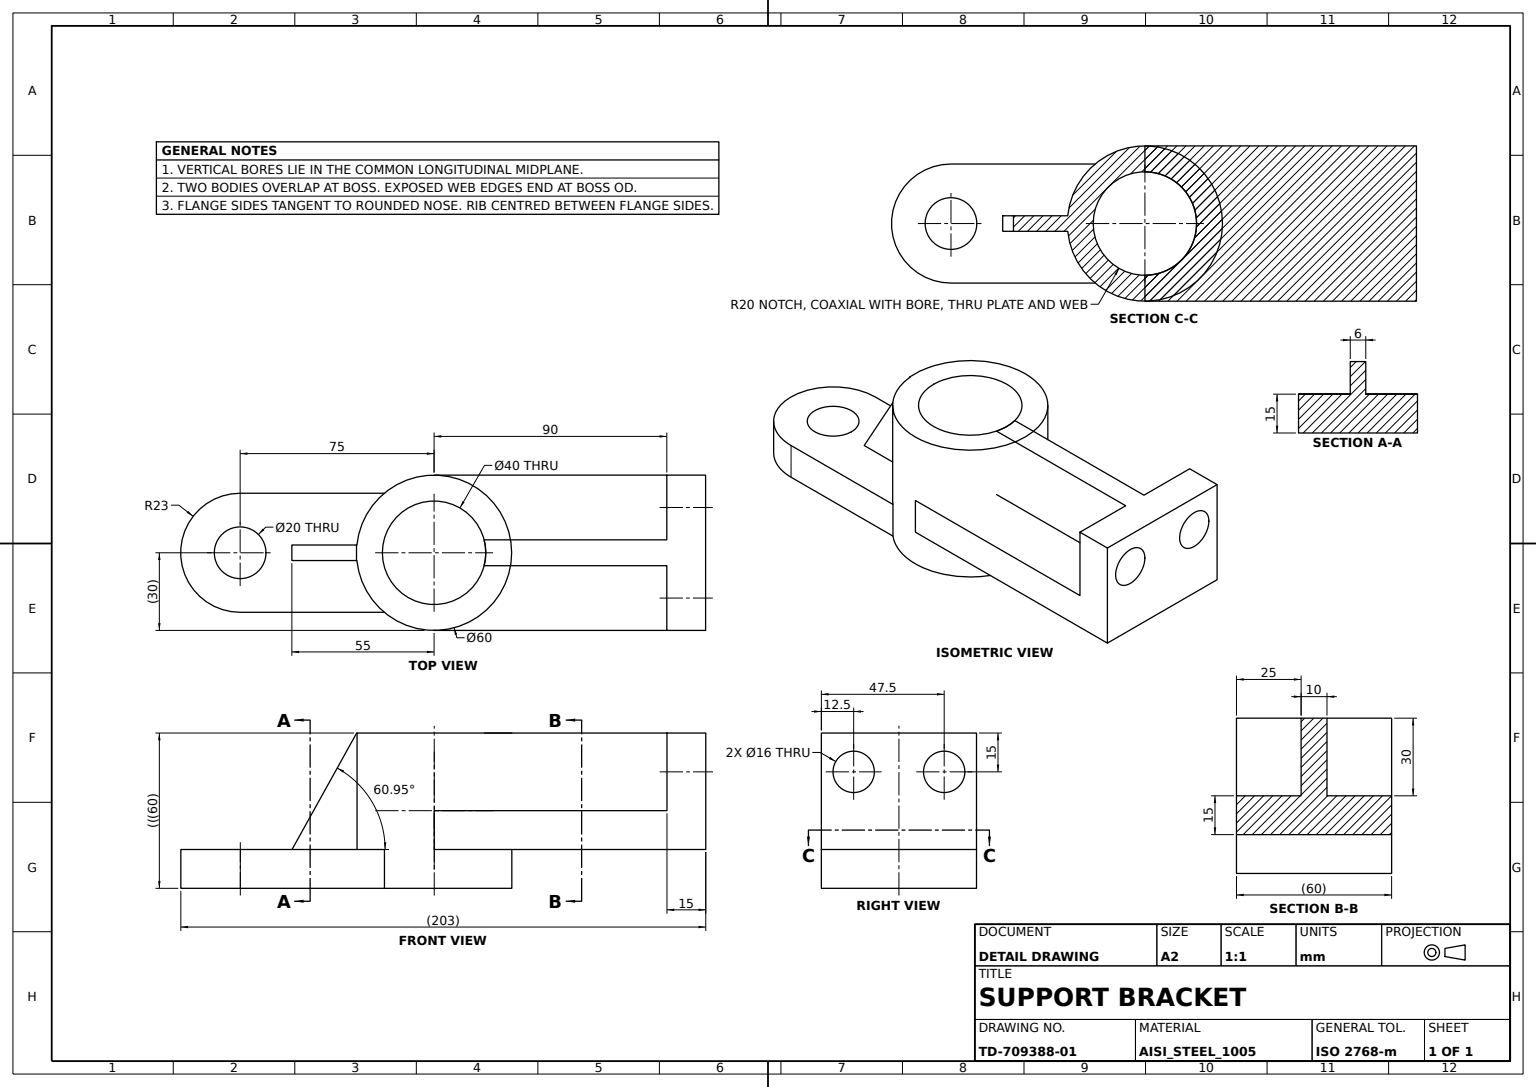
ISO-10303-21;
HEADER;
FILE_DESCRIPTION((''),'2;1');
FILE_NAME('','',(''),(''),'','','');
FILE_SCHEMA(('AUTOMOTIVE_DESIGN'));
ENDSEC;
DATA;
#1=APPLICATION_CONTEXT('');
#2=PRODUCT_CONTEXT('',#1,'mechanical');
#3=PRODUCT('','','',(#2));
#4=PRODUCT_DEFINITION_FORMATION('','',#3);
#5=PRODUCT_DEFINITION_CONTEXT('',#1,'design');
#6=PRODUCT_DEFINITION('','',#4,#5);
#7=PRODUCT_DEFINITION_SHAPE('','',#6);
#8=(LENGTH_UNIT()NAMED_UNIT(*)SI_UNIT(.MILLI.,.METRE.));
#9=(NAMED_UNIT(*)PLANE_ANGLE_UNIT()SI_UNIT($,.RADIAN.));
#10=(NAMED_UNIT(*)SI_UNIT($,.STERADIAN.)SOLID_ANGLE_UNIT());
#11=UNCERTAINTY_MEASURE_WITH_UNIT(LENGTH_MEASURE(0.005),#8,'distance_accuracy_value','');
#12=(GEOMETRIC_REPRESENTATION_CONTEXT(3)GLOBAL_UNCERTAINTY_ASSIGNED_CONTEXT((#11))GLOBAL_UNIT_ASSIGNED_CONTEXT((#8,#9,#10))REPRESENTATION_CONTEXT('',''));
#13=CARTESIAN_POINT('',(85.,0.,0.));
#14=VERTEX_POINT('',#13);
#15=CARTESIAN_POINT('',(75.,0.,0.));
#16=DIRECTION('',(0.,0.,1.));
#17=DIRECTION('',(1.,0.,0.));
#18=AXIS2_PLACEMENT_3D('',#15,#16,#17);
#19=CIRCLE('',#18,10.);
#20=EDGE_CURVE('',#14,#14,#19,.T.);
#21=ORIENTED_EDGE('',*,*,#20,.T.);
#22=EDGE_LOOP('',(#21));
#23=FACE_BOUND('',#22,.T.);
#24=CARTESIAN_POINT('',(20.,0.,0.));
#25=VERTEX_POINT('',#24);
#26=CARTESIAN_POINT('',(0.,0.,0.));
#27=AXIS2_PLACEMENT_3D('',#26,#16,#17);
#28=CIRCLE('',#27,20.);
#29=EDGE_CURVE('',#25,#25,#28,.T.);
#30=ORIENTED_EDGE('',*,*,#29,.T.);
#31=EDGE_LOOP('',(#30));
#32=FACE_BOUND('',#31,.T.);
#33=CARTESIAN_POINT('',(19.26136,-23.,0.));
#34=VERTEX_POINT('',#33);
#35=CARTESIAN_POINT('',(75.,-23.,0.));
#36=VERTEX_POINT('',#35);
#37=VECTOR('',#17,1000.);
#38=LINE('',#33,#37);
#39=EDGE_CURVE('',#34,#36,#38,.T.);
#40=ORIENTED_EDGE('',*,*,#39,.F.);
#41=CARTESIAN_POINT('',(19.26136,23.,0.));
#42=VERTEX_POINT('',#41);
#43=CIRCLE('',#27,30.);
#44=EDGE_CURVE('',#42,#34,#43,.T.);
#45=ORIENTED_EDGE('',*,*,#44,.F.);
#46=CARTESIAN_POINT('',(75.,23.,0.));
#47=VERTEX_POINT('',#46);
#48=DIRECTION('',(-1.,0.,0.));
#49=VECTOR('',#48,1000.);
#50=LINE('',#46,#49);
#51=EDGE_CURVE('',#47,#42,#50,.T.);
#52=ORIENTED_EDGE('',*,*,#51,.F.);
#53=CIRCLE('',#18,23.);
#54=EDGE_CURVE('',#36,#47,#53,.T.);
#55=ORIENTED_EDGE('',*,*,#54,.F.);
#56=EDGE_LOOP('',(#40,#45,#52,#55));
#57=FACE_BOUND('',#56,.T.);
#58=PLANE('',#27);
#59=ADVANCED_FACE('',(#23,#32,#57),#58,.F.);
#60=CARTESIAN_POINT('',(75.,23.,15.));
#61=VERTEX_POINT('',#60);
#62=DIRECTION('',(0.,0.,-1.));
#63=VECTOR('',#62,1000.);
#64=LINE('',#60,#63);
#65=EDGE_CURVE('',#61,#47,#64,.T.);
#66=ORIENTED_EDGE('',*,*,#65,.T.);
#67=ORIENTED_EDGE('',*,*,#51,.T.);
#68=CARTESIAN_POINT('',(19.26136,23.,15.));
#69=VERTEX_POINT('',#68);
#70=LINE('',#68,#63);
#71=EDGE_CURVE('',#69,#42,#70,.T.);
#72=ORIENTED_EDGE('',*,*,#71,.F.);
#73=LINE('',#60,#49);
#74=EDGE_CURVE('',#61,#69,#73,.T.);
#75=ORIENTED_EDGE('',*,*,#74,.F.);
#76=EDGE_LOOP('',(#66,#67,#72,#75));
#77=FACE_BOUND('',#76,.T.);
#78=DIRECTION('',(0.,-1.,0.));
#79=AXIS2_PLACEMENT_3D('',#60,#78,#62);
#80=PLANE('',#79);
#81=ADVANCED_FACE('',(#77),#80,.F.);
#82=CARTESIAN_POINT('',(29.849623,3.,15.));
#83=VERTEX_POINT('',#82);
#84=CARTESIAN_POINT('',(55.,3.,15.));
#85=VERTEX_POINT('',#84);
#86=CARTESIAN_POINT('',(0.,3.,15.));
#87=LINE('',#86,#49);
#88=EDGE_CURVE('',#83,#85,#87,.F.);
#89=ORIENTED_EDGE('',*,*,#88,.F.);
#90=CARTESIAN_POINT('',(29.849623,3.,60.));
#91=VERTEX_POINT('',#90);
#92=LINE('',#90,#63);
#93=EDGE_CURVE('',#91,#83,#92,.T.);
#94=ORIENTED_EDGE('',*,*,#93,.F.);
#95=CARTESIAN_POINT('',(30.,3.,60.));
#96=VERTEX_POINT('',#95);
#97=CARTESIAN_POINT('',(26.5,3.,60.));
#98=LINE('',#97,#37);
#99=EDGE_CURVE('',#91,#96,#98,.T.);
#100=ORIENTED_EDGE('',*,*,#99,.T.);
#101=DIRECTION('',(0.485642931,0.,-0.874157276));
#102=VECTOR('',#101,1000.);
#103=LINE('',#95,#102);
#104=EDGE_CURVE('',#96,#85,#103,.T.);
#105=ORIENTED_EDGE('',*,*,#104,.T.);
#106=EDGE_LOOP('',(#89,#94,#100,#105));
#107=FACE_BOUND('',#106,.T.);
#108=CARTESIAN_POINT('',(0.,3.,0.));
#109=DIRECTION('',(0.,1.,0.));
#110=AXIS2_PLACEMENT_3D('',#108,#109,#16);
#111=PLANE('',#110);
#112=ADVANCED_FACE('',(#107),#111,.T.);
#113=CARTESIAN_POINT('',(29.849623,-3.,15.));
#114=VERTEX_POINT('',#113);
#115=CARTESIAN_POINT('',(29.849623,-3.,60.));
#116=VERTEX_POINT('',#115);
#117=LINE('',#115,#63);
#118=EDGE_CURVE('',#114,#116,#117,.F.);
#119=ORIENTED_EDGE('',*,*,#118,.F.);
#120=CARTESIAN_POINT('',(55.,-3.,15.));
#121=VERTEX_POINT('',#120);
#122=CARTESIAN_POINT('',(0.,-3.,15.));
#123=LINE('',#122,#49);
#124=EDGE_CURVE('',#121,#114,#123,.T.);
#125=ORIENTED_EDGE('',*,*,#124,.F.);
#126=CARTESIAN_POINT('',(30.,-3.,60.));
#127=VERTEX_POINT('',#126);
#128=LINE('',#126,#102);
#129=EDGE_CURVE('',#127,#121,#128,.T.);
#130=ORIENTED_EDGE('',*,*,#129,.F.);
#131=CARTESIAN_POINT('',(26.5,-3.,60.));
#132=LINE('',#131,#37);
#133=EDGE_CURVE('',#116,#127,#132,.T.);
#134=ORIENTED_EDGE('',*,*,#133,.F.);
#135=EDGE_LOOP('',(#119,#125,#130,#134));
#136=FACE_BOUND('',#135,.T.);
#137=CARTESIAN_POINT('',(0.,-3.,0.));
#138=AXIS2_PLACEMENT_3D('',#137,#109,#16);
#139=PLANE('',#138);
#140=ADVANCED_FACE('',(#136),#139,.F.);
#141=VECTOR('',#109,1000.);
#142=LINE('',#126,#141);
#143=EDGE_CURVE('',#127,#96,#142,.T.);
#144=ORIENTED_EDGE('',*,*,#143,.T.);
#145=ORIENTED_EDGE('',*,*,#99,.F.);
#146=CARTESIAN_POINT('',(0.,0.,60.));
#147=AXIS2_PLACEMENT_3D('',#146,#16,#17);
#148=CIRCLE('',#147,30.);
#149=EDGE_CURVE('',#91,#116,#148,.T.);
#150=ORIENTED_EDGE('',*,*,#149,.T.);
#151=ORIENTED_EDGE('',*,*,#133,.T.);
#152=EDGE_LOOP('',(#144,#145,#150,#151));
#153=FACE_BOUND('',#152,.T.);
#154=CARTESIAN_POINT('',(20.,0.,60.));
#155=VERTEX_POINT('',#154);
#156=CIRCLE('',#147,20.);
#157=EDGE_CURVE('',#155,#155,#156,.T.);
#158=ORIENTED_EDGE('',*,*,#157,.F.);
#159=EDGE_LOOP('',(#158));
#160=FACE_BOUND('',#159,.T.);
#161=PLANE('',#147);
#162=ADVANCED_FACE('',(#153,#160),#161,.T.);
#163=CARTESIAN_POINT('',(75.,-23.,15.));
#164=VERTEX_POINT('',#163);
#165=LINE('',#163,#63);
#166=EDGE_CURVE('',#164,#36,#165,.T.);
#167=ORIENTED_EDGE('',*,*,#166,.F.);
#168=CARTESIAN_POINT('',(19.26136,-23.,15.));
#169=VERTEX_POINT('',#168);
#170=LINE('',#168,#37);
#171=EDGE_CURVE('',#169,#164,#170,.T.);
#172=ORIENTED_EDGE('',*,*,#171,.F.);
#173=LINE('',#168,#63);
#174=EDGE_CURVE('',#169,#34,#173,.T.);
#175=ORIENTED_EDGE('',*,*,#174,.T.);
#176=ORIENTED_EDGE('',*,*,#39,.T.);
#177=EDGE_LOOP('',(#167,#172,#175,#176));
#178=FACE_BOUND('',#177,.T.);
#179=AXIS2_PLACEMENT_3D('',#168,#109,#16);
#180=PLANE('',#179);
#181=ADVANCED_FACE('',(#178),#180,.F.);
#182=ORIENTED_EDGE('',*,*,#54,.T.);
#183=ORIENTED_EDGE('',*,*,#65,.F.);
#184=CARTESIAN_POINT('',(75.,0.,15.));
#185=AXIS2_PLACEMENT_3D('',#184,#16,#17);
#186=CIRCLE('',#185,23.);
#187=EDGE_CURVE('',#164,#61,#186,.T.);
#188=ORIENTED_EDGE('',*,*,#187,.F.);
#189=ORIENTED_EDGE('',*,*,#166,.T.);
#190=EDGE_LOOP('',(#182,#183,#188,#189));
#191=FACE_BOUND('',#190,.T.);
#192=AXIS2_PLACEMENT_3D('',#184,#62,#48);
#193=CYLINDRICAL_SURFACE('',#192,23.);
#194=ADVANCED_FACE('',(#191),#193,.T.);
#195=CARTESIAN_POINT('',(0.,0.,15.));
#196=AXIS2_PLACEMENT_3D('',#195,#62,#17);
#197=CIRCLE('',#196,30.);
#198=EDGE_CURVE('',#69,#83,#197,.T.);
#199=ORIENTED_EDGE('',*,*,#198,.F.);
#200=ORIENTED_EDGE('',*,*,#71,.T.);
#201=ORIENTED_EDGE('',*,*,#44,.T.);
#202=ORIENTED_EDGE('',*,*,#174,.F.);
#203=EDGE_CURVE('',#114,#169,#197,.T.);
#204=ORIENTED_EDGE('',*,*,#203,.F.);
#205=ORIENTED_EDGE('',*,*,#118,.T.);
#206=ORIENTED_EDGE('',*,*,#149,.F.);
#207=ORIENTED_EDGE('',*,*,#93,.T.);
#208=EDGE_LOOP('',(#199,#200,#201,#202,#204,#205,#206,#207));
#209=FACE_BOUND('',#208,.T.);
#210=AXIS2_PLACEMENT_3D('',#146,#62,#48);
#211=CYLINDRICAL_SURFACE('',#210,30.);
#212=ADVANCED_FACE('',(#209),#211,.T.);
#213=ORIENTED_EDGE('',*,*,#157,.T.);
#214=EDGE_LOOP('',(#213));
#215=FACE_BOUND('',#214,.T.);
#216=ORIENTED_EDGE('',*,*,#29,.F.);
#217=EDGE_LOOP('',(#216));
#218=FACE_BOUND('',#217,.T.);
#219=CYLINDRICAL_SURFACE('',#210,20.);
#220=ADVANCED_FACE('',(#215,#218),#219,.F.);
#221=ORIENTED_EDGE('',*,*,#20,.F.);
#222=EDGE_LOOP('',(#221));
#223=FACE_BOUND('',#222,.T.);
#224=CARTESIAN_POINT('',(65.,0.,15.));
#225=VERTEX_POINT('',#224);
#226=CIRCLE('',#192,10.);
#227=EDGE_CURVE('',#225,#225,#226,.F.);
#228=ORIENTED_EDGE('',*,*,#227,.T.);
#229=EDGE_LOOP('',(#228));
#230=FACE_BOUND('',#229,.T.);
#231=CARTESIAN_POINT('',(75.,0.,60.));
#232=AXIS2_PLACEMENT_3D('',#231,#62,#48);
#233=CYLINDRICAL_SURFACE('',#232,10.);
#234=ADVANCED_FACE('',(#223,#230),#233,.F.);
#235=ORIENTED_EDGE('',*,*,#203,.T.);
#236=ORIENTED_EDGE('',*,*,#171,.T.);
#237=ORIENTED_EDGE('',*,*,#187,.T.);
#238=ORIENTED_EDGE('',*,*,#74,.T.);
#239=ORIENTED_EDGE('',*,*,#198,.T.);
#240=ORIENTED_EDGE('',*,*,#88,.T.);
#241=LINE('',#120,#141);
#242=EDGE_CURVE('',#85,#121,#241,.F.);
#243=ORIENTED_EDGE('',*,*,#242,.T.);
#244=ORIENTED_EDGE('',*,*,#124,.T.);
#245=EDGE_LOOP('',(#235,#236,#237,#238,#239,#240,#243,#244));
#246=FACE_BOUND('',#245,.T.);
#247=ORIENTED_EDGE('',*,*,#227,.F.);
#248=EDGE_LOOP('',(#247));
#249=FACE_BOUND('',#248,.T.);
#250=AXIS2_PLACEMENT_3D('',#195,#62,#48);
#251=PLANE('',#250);
#252=ADVANCED_FACE('',(#246,#249),#251,.F.);
#253=ORIENTED_EDGE('',*,*,#143,.F.);
#254=ORIENTED_EDGE('',*,*,#129,.T.);
#255=ORIENTED_EDGE('',*,*,#242,.F.);
#256=ORIENTED_EDGE('',*,*,#104,.F.);
#257=EDGE_LOOP('',(#253,#254,#255,#256));
#258=FACE_BOUND('',#257,.T.);
#259=DIRECTION('',(0.874157276,0.,0.485642931));
#260=AXIS2_PLACEMENT_3D('',#126,#259,#101);
#261=PLANE('',#260);
#262=ADVANCED_FACE('',(#258),#261,.T.);
#263=CLOSED_SHELL('',(#59,#81,#112,#140,#162,#181,#194,#212,#220,#234,#252,#262));
#264=MANIFOLD_SOLID_BREP('',#263);
#265=CARTESIAN_POINT('',(-90.,5.,60.));
#266=VERTEX_POINT('',#265);
#267=CARTESIAN_POINT('',(-90.,30.,60.));
#268=VERTEX_POINT('',#267);
#269=CARTESIAN_POINT('',(-90.,-30.,60.));
#270=LINE('',#269,#141);
#271=EDGE_CURVE('',#266,#268,#270,.T.);
#272=ORIENTED_EDGE('',*,*,#271,.F.);
#273=CARTESIAN_POINT('',(-90.,5.,30.));
#274=VERTEX_POINT('',#273);
#275=LINE('',#265,#63);
#276=EDGE_CURVE('',#266,#274,#275,.T.);
#277=ORIENTED_EDGE('',*,*,#276,.T.);
#278=CARTESIAN_POINT('',(-90.,30.,30.));
#279=VERTEX_POINT('',#278);
#280=CARTESIAN_POINT('',(-90.,-30.,30.));
#281=LINE('',#280,#141);
#282=EDGE_CURVE('',#274,#279,#281,.T.);
#283=ORIENTED_EDGE('',*,*,#282,.T.);
#284=VECTOR('',#16,1000.);
#285=LINE('',#278,#284);
#286=EDGE_CURVE('',#279,#268,#285,.T.);
#287=ORIENTED_EDGE('',*,*,#286,.T.);
#288=EDGE_LOOP('',(#272,#277,#283,#287));
#289=FACE_BOUND('',#288,.T.);
#290=CARTESIAN_POINT('',(-90.,17.5,53.));
#291=VERTEX_POINT('',#290);
#292=CARTESIAN_POINT('',(-90.,17.5,45.));
#293=AXIS2_PLACEMENT_3D('',#292,#48,#16);
#294=CIRCLE('',#293,8.);
#295=EDGE_CURVE('',#291,#291,#294,.T.);
#296=ORIENTED_EDGE('',*,*,#295,.T.);
#297=EDGE_LOOP('',(#296));
#298=FACE_BOUND('',#297,.T.);
#299=AXIS2_PLACEMENT_3D('',#280,#48,#16);
#300=PLANE('',#299);
#301=ADVANCED_FACE('',(#289,#298),#300,.F.);
#302=CARTESIAN_POINT('',(0.,20.,30.));
#303=VERTEX_POINT('',#302);
#304=CARTESIAN_POINT('',(0.,30.,30.));
#305=VERTEX_POINT('',#304);
#306=CARTESIAN_POINT('',(0.,-30.,30.));
#307=LINE('',#306,#141);
#308=EDGE_CURVE('',#303,#305,#307,.T.);
#309=ORIENTED_EDGE('',*,*,#308,.F.);
#310=CARTESIAN_POINT('',(0.,20.,15.));
#311=VERTEX_POINT('',#310);
#312=CARTESIAN_POINT('',(0.,20.,66.));
#313=LINE('',#312,#63);
#314=EDGE_CURVE('',#311,#303,#313,.F.);
#315=ORIENTED_EDGE('',*,*,#314,.F.);
#316=CARTESIAN_POINT('',(0.,30.,15.));
#317=VERTEX_POINT('',#316);
#318=CARTESIAN_POINT('',(0.,-30.,15.));
#319=LINE('',#318,#141);
#320=EDGE_CURVE('',#311,#317,#319,.T.);
#321=ORIENTED_EDGE('',*,*,#320,.T.);
#322=LINE('',#316,#284);
#323=EDGE_CURVE('',#317,#305,#322,.T.);
#324=ORIENTED_EDGE('',*,*,#323,.T.);
#325=EDGE_LOOP('',(#309,#315,#321,#324));
#326=FACE_BOUND('',#325,.T.);
#327=AXIS2_PLACEMENT_3D('',#318,#48,#16);
#328=PLANE('',#327);
#329=ADVANCED_FACE('',(#326),#328,.F.);
#330=ORIENTED_EDGE('',*,*,#308,.T.);
#331=CARTESIAN_POINT('',(-30.,30.,30.));
#332=LINE('',#331,#49);
#333=EDGE_CURVE('',#305,#279,#332,.T.);
#334=ORIENTED_EDGE('',*,*,#333,.T.);
#335=ORIENTED_EDGE('',*,*,#282,.F.);
#336=CARTESIAN_POINT('',(-19.364917,5.,30.));
#337=VERTEX_POINT('',#336);
#338=LINE('',#273,#37);
#339=EDGE_CURVE('',#274,#337,#338,.T.);
#340=ORIENTED_EDGE('',*,*,#339,.T.);
#341=CARTESIAN_POINT('',(0.,0.,30.));
#342=AXIS2_PLACEMENT_3D('',#341,#62,#48);
#343=CIRCLE('',#342,20.);
#344=EDGE_CURVE('',#303,#337,#343,.F.);
#345=ORIENTED_EDGE('',*,*,#344,.F.);
#346=EDGE_LOOP('',(#330,#334,#335,#340,#345));
#347=FACE_BOUND('',#346,.T.);
#348=CARTESIAN_POINT('',(-30.,-30.,30.));
#349=AXIS2_PLACEMENT_3D('',#348,#62,#48);
#350=PLANE('',#349);
#351=ADVANCED_FACE('',(#347),#350,.F.);
#352=CARTESIAN_POINT('',(-105.,30.,60.));
#353=VERTEX_POINT('',#352);
#354=LINE('',#267,#49);
#355=EDGE_CURVE('',#268,#353,#354,.T.);
#356=ORIENTED_EDGE('',*,*,#355,.F.);
#357=ORIENTED_EDGE('',*,*,#286,.F.);
#358=ORIENTED_EDGE('',*,*,#333,.F.);
#359=ORIENTED_EDGE('',*,*,#323,.F.);
#360=CARTESIAN_POINT('',(-105.,30.,15.));
#361=VERTEX_POINT('',#360);
#362=LINE('',#360,#37);
#363=EDGE_CURVE('',#361,#317,#362,.T.);
#364=ORIENTED_EDGE('',*,*,#363,.F.);
#365=CARTESIAN_POINT('',(-105.,30.,30.));
#366=LINE('',#365,#63);
#367=EDGE_CURVE('',#353,#361,#366,.T.);
#368=ORIENTED_EDGE('',*,*,#367,.F.);
#369=EDGE_LOOP('',(#356,#357,#358,#359,#364,#368));
#370=FACE_BOUND('',#369,.T.);
#371=CARTESIAN_POINT('',(0.,30.,0.));
#372=AXIS2_PLACEMENT_3D('',#371,#78,#62);
#373=PLANE('',#372);
#374=ADVANCED_FACE('',(#370),#373,.F.);
#375=VERTEX_POINT('',#306);
#376=VERTEX_POINT('',#280);
#377=LINE('',#348,#49);
#378=EDGE_CURVE('',#375,#376,#377,.T.);
#379=ORIENTED_EDGE('',*,*,#378,.T.);
#380=VERTEX_POINT('',#269);
#381=LINE('',#280,#284);
#382=EDGE_CURVE('',#376,#380,#381,.T.);
#383=ORIENTED_EDGE('',*,*,#382,.T.);
#384=CARTESIAN_POINT('',(-105.,-30.,60.));
#385=VERTEX_POINT('',#384);
#386=LINE('',#269,#49);
#387=EDGE_CURVE('',#380,#385,#386,.T.);
#388=ORIENTED_EDGE('',*,*,#387,.T.);
#389=CARTESIAN_POINT('',(-105.,-30.,15.));
#390=VERTEX_POINT('',#389);
#391=LINE('',#384,#63);
#392=EDGE_CURVE('',#385,#390,#391,.T.);
#393=ORIENTED_EDGE('',*,*,#392,.T.);
#394=VERTEX_POINT('',#318);
#395=LINE('',#389,#37);
#396=EDGE_CURVE('',#390,#394,#395,.T.);
#397=ORIENTED_EDGE('',*,*,#396,.T.);
#398=LINE('',#318,#284);
#399=EDGE_CURVE('',#394,#375,#398,.T.);
#400=ORIENTED_EDGE('',*,*,#399,.T.);
#401=EDGE_LOOP('',(#379,#383,#388,#393,#397,#400));
#402=FACE_BOUND('',#401,.T.);
#403=CARTESIAN_POINT('',(0.,-30.,0.));
#404=AXIS2_PLACEMENT_3D('',#403,#78,#62);
#405=PLANE('',#404);
#406=ADVANCED_FACE('',(#402),#405,.T.);
#407=ORIENTED_EDGE('',*,*,#387,.F.);
#408=CARTESIAN_POINT('',(-90.,-5.,60.));
#409=VERTEX_POINT('',#408);
#410=EDGE_CURVE('',#380,#409,#270,.T.);
#411=ORIENTED_EDGE('',*,*,#410,.T.);
#412=CARTESIAN_POINT('',(-19.364917,-5.,60.));
#413=VERTEX_POINT('',#412);
#414=CARTESIAN_POINT('',(-30.,-5.,60.));
#415=LINE('',#414,#49);
#416=EDGE_CURVE('',#413,#409,#415,.T.);
#417=ORIENTED_EDGE('',*,*,#416,.F.);
#418=CARTESIAN_POINT('',(-19.364917,5.,60.));
#419=VERTEX_POINT('',#418);
#420=AXIS2_PLACEMENT_3D('',#146,#62,#17);
#421=CIRCLE('',#420,20.);
#422=EDGE_CURVE('',#413,#419,#421,.T.);
#423=ORIENTED_EDGE('',*,*,#422,.T.);
#424=CARTESIAN_POINT('',(-30.,5.,60.));
#425=LINE('',#424,#49);
#426=EDGE_CURVE('',#419,#266,#425,.T.);
#427=ORIENTED_EDGE('',*,*,#426,.T.);
#428=ORIENTED_EDGE('',*,*,#271,.T.);
#429=ORIENTED_EDGE('',*,*,#355,.T.);
#430=LINE('',#384,#141);
#431=EDGE_CURVE('',#385,#353,#430,.T.);
#432=ORIENTED_EDGE('',*,*,#431,.F.);
#433=EDGE_LOOP('',(#407,#411,#417,#423,#427,#428,#429,#432));
#434=FACE_BOUND('',#433,.T.);
#435=AXIS2_PLACEMENT_3D('',#269,#62,#48);
#436=PLANE('',#435);
#437=ADVANCED_FACE('',(#434),#436,.F.);
#438=CARTESIAN_POINT('',(-90.,-5.,30.));
#439=VERTEX_POINT('',#438);
#440=CARTESIAN_POINT('',(-19.364917,-5.,30.));
#441=VERTEX_POINT('',#440);
#442=LINE('',#438,#37);
#443=EDGE_CURVE('',#439,#441,#442,.T.);
#444=ORIENTED_EDGE('',*,*,#443,.T.);
#445=LINE('',#412,#63);
#446=EDGE_CURVE('',#413,#441,#445,.T.);
#447=ORIENTED_EDGE('',*,*,#446,.F.);
#448=ORIENTED_EDGE('',*,*,#416,.T.);
#449=LINE('',#408,#63);
#450=EDGE_CURVE('',#409,#439,#449,.T.);
#451=ORIENTED_EDGE('',*,*,#450,.T.);
#452=EDGE_LOOP('',(#444,#447,#448,#451));
#453=FACE_BOUND('',#452,.T.);
#454=CARTESIAN_POINT('',(0.,-5.,0.));
#455=AXIS2_PLACEMENT_3D('',#454,#78,#62);
#456=PLANE('',#455);
#457=ADVANCED_FACE('',(#453),#456,.T.);
#458=CARTESIAN_POINT('',(-105.,9.5,45.));
#459=VERTEX_POINT('',#458);
#460=CARTESIAN_POINT('',(-105.,17.5,45.));
#461=AXIS2_PLACEMENT_3D('',#460,#48,#78);
#462=CIRCLE('',#461,8.);
#463=EDGE_CURVE('',#459,#459,#462,.T.);
#464=ORIENTED_EDGE('',*,*,#463,.T.);
#465=EDGE_LOOP('',(#464));
#466=FACE_BOUND('',#465,.T.);
#467=ORIENTED_EDGE('',*,*,#295,.F.);
#468=EDGE_LOOP('',(#467));
#469=FACE_BOUND('',#468,.T.);
#470=CARTESIAN_POINT('',(-85.,17.5,45.));
#471=AXIS2_PLACEMENT_3D('',#470,#48,#16);
#472=CYLINDRICAL_SURFACE('',#471,8.);
#473=ADVANCED_FACE('',(#466,#469),#472,.F.);
#474=CARTESIAN_POINT('',(-90.,-17.5,53.));
#475=VERTEX_POINT('',#474);
#476=CARTESIAN_POINT('',(-90.,-17.5,45.));
#477=AXIS2_PLACEMENT_3D('',#476,#48,#16);
#478=CIRCLE('',#477,8.);
#479=EDGE_CURVE('',#475,#475,#478,.T.);
#480=ORIENTED_EDGE('',*,*,#479,.T.);
#481=EDGE_LOOP('',(#480));
#482=FACE_BOUND('',#481,.T.);
#483=ORIENTED_EDGE('',*,*,#450,.F.);
#484=ORIENTED_EDGE('',*,*,#410,.F.);
#485=ORIENTED_EDGE('',*,*,#382,.F.);
#486=EDGE_CURVE('',#376,#439,#281,.T.);
#487=ORIENTED_EDGE('',*,*,#486,.T.);
#488=EDGE_LOOP('',(#483,#484,#485,#487));
#489=FACE_BOUND('',#488,.T.);
#490=ADVANCED_FACE('',(#482,#489),#300,.F.);
#491=ORIENTED_EDGE('',*,*,#443,.F.);
#492=ORIENTED_EDGE('',*,*,#486,.F.);
#493=ORIENTED_EDGE('',*,*,#378,.F.);
#494=CARTESIAN_POINT('',(0.,-20.,30.));
#495=VERTEX_POINT('',#494);
#496=EDGE_CURVE('',#375,#495,#307,.T.);
#497=ORIENTED_EDGE('',*,*,#496,.T.);
#498=EDGE_CURVE('',#441,#495,#343,.F.);
#499=ORIENTED_EDGE('',*,*,#498,.F.);
#500=EDGE_LOOP('',(#491,#492,#493,#497,#499));
#501=FACE_BOUND('',#500,.T.);
#502=ADVANCED_FACE('',(#501),#350,.F.);
#503=ORIENTED_EDGE('',*,*,#367,.T.);
#504=LINE('',#389,#141);
#505=EDGE_CURVE('',#390,#361,#504,.T.);
#506=ORIENTED_EDGE('',*,*,#505,.F.);
#507=ORIENTED_EDGE('',*,*,#392,.F.);
#508=ORIENTED_EDGE('',*,*,#431,.T.);
#509=EDGE_LOOP('',(#503,#506,#507,#508));
#510=FACE_BOUND('',#509,.T.);
#511=CARTESIAN_POINT('',(-105.,-25.5,45.));
#512=VERTEX_POINT('',#511);
#513=CARTESIAN_POINT('',(-105.,-17.5,45.));
#514=AXIS2_PLACEMENT_3D('',#513,#48,#78);
#515=CIRCLE('',#514,8.);
#516=EDGE_CURVE('',#512,#512,#515,.T.);
#517=ORIENTED_EDGE('',*,*,#516,.F.);
#518=EDGE_LOOP('',(#517));
#519=FACE_BOUND('',#518,.T.);
#520=ORIENTED_EDGE('',*,*,#463,.F.);
#521=EDGE_LOOP('',(#520));
#522=FACE_BOUND('',#521,.T.);
#523=CARTESIAN_POINT('',(-105.,-30.,30.));
#524=AXIS2_PLACEMENT_3D('',#523,#17,#62);
#525=PLANE('',#524);
#526=ADVANCED_FACE('',(#510,#519,#522),#525,.F.);
#527=ORIENTED_EDGE('',*,*,#363,.T.);
#528=ORIENTED_EDGE('',*,*,#320,.F.);
#529=CARTESIAN_POINT('',(0.,-20.,15.));
#530=VERTEX_POINT('',#529);
#531=AXIS2_PLACEMENT_3D('',#195,#16,#17);
#532=CIRCLE('',#531,20.);
#533=EDGE_CURVE('',#530,#311,#532,.F.);
#534=ORIENTED_EDGE('',*,*,#533,.F.);
#535=EDGE_CURVE('',#394,#530,#319,.T.);
#536=ORIENTED_EDGE('',*,*,#535,.F.);
#537=ORIENTED_EDGE('',*,*,#396,.F.);
#538=ORIENTED_EDGE('',*,*,#505,.T.);
#539=EDGE_LOOP('',(#527,#528,#534,#536,#537,#538));
#540=FACE_BOUND('',#539,.T.);
#541=AXIS2_PLACEMENT_3D('',#389,#16,#17);
#542=PLANE('',#541);
#543=ADVANCED_FACE('',(#540),#542,.F.);
#544=ORIENTED_EDGE('',*,*,#399,.F.);
#545=ORIENTED_EDGE('',*,*,#535,.T.);
#546=CARTESIAN_POINT('',(0.,-20.,66.));
#547=LINE('',#546,#63);
#548=EDGE_CURVE('',#495,#530,#547,.T.);
#549=ORIENTED_EDGE('',*,*,#548,.F.);
#550=ORIENTED_EDGE('',*,*,#496,.F.);
#551=EDGE_LOOP('',(#544,#545,#549,#550));
#552=FACE_BOUND('',#551,.T.);
#553=ADVANCED_FACE('',(#552),#328,.F.);
#554=ORIENTED_EDGE('',*,*,#516,.T.);
#555=EDGE_LOOP('',(#554));
#556=FACE_BOUND('',#555,.T.);
#557=ORIENTED_EDGE('',*,*,#479,.F.);
#558=EDGE_LOOP('',(#557));
#559=FACE_BOUND('',#558,.T.);
#560=CARTESIAN_POINT('',(-85.,-17.5,45.));
#561=AXIS2_PLACEMENT_3D('',#560,#48,#16);
#562=CYLINDRICAL_SURFACE('',#561,8.);
#563=ADVANCED_FACE('',(#556,#559),#562,.F.);
#564=LINE('',#418,#63);
#565=EDGE_CURVE('',#419,#337,#564,.T.);
#566=ORIENTED_EDGE('',*,*,#565,.T.);
#567=ORIENTED_EDGE('',*,*,#339,.F.);
#568=ORIENTED_EDGE('',*,*,#276,.F.);
#569=ORIENTED_EDGE('',*,*,#426,.F.);
#570=EDGE_LOOP('',(#566,#567,#568,#569));
#571=FACE_BOUND('',#570,.T.);
#572=CARTESIAN_POINT('',(0.,5.,0.));
#573=AXIS2_PLACEMENT_3D('',#572,#78,#62);
#574=PLANE('',#573);
#575=ADVANCED_FACE('',(#571),#574,.F.);
#576=ORIENTED_EDGE('',*,*,#498,.T.);
#577=ORIENTED_EDGE('',*,*,#548,.T.);
#578=ORIENTED_EDGE('',*,*,#533,.T.);
#579=ORIENTED_EDGE('',*,*,#314,.T.);
#580=ORIENTED_EDGE('',*,*,#344,.T.);
#581=ORIENTED_EDGE('',*,*,#565,.F.);
#582=ORIENTED_EDGE('',*,*,#422,.F.);
#583=ORIENTED_EDGE('',*,*,#446,.T.);
#584=EDGE_LOOP('',(#576,#577,#578,#579,#580,#581,#582,#583));
#585=FACE_BOUND('',#584,.T.);
#586=CARTESIAN_POINT('',(0.,0.,66.));
#587=AXIS2_PLACEMENT_3D('',#586,#62,#48);
#588=CYLINDRICAL_SURFACE('',#587,20.);
#589=ADVANCED_FACE('',(#585),#588,.F.);
#590=CLOSED_SHELL('',(#301,#329,#351,#374,#406,#437,#457,#473,#490,#502,#526,#543,#553,#563,#575,#589));
#591=MANIFOLD_SOLID_BREP('',#590);
#592=ADVANCED_BREP_SHAPE_REPRESENTATION('',(#264,#591),#12);
#593=SHAPE_DEFINITION_REPRESENTATION(#7,#592);
ENDSEC;
END-ISO-10303-21;
